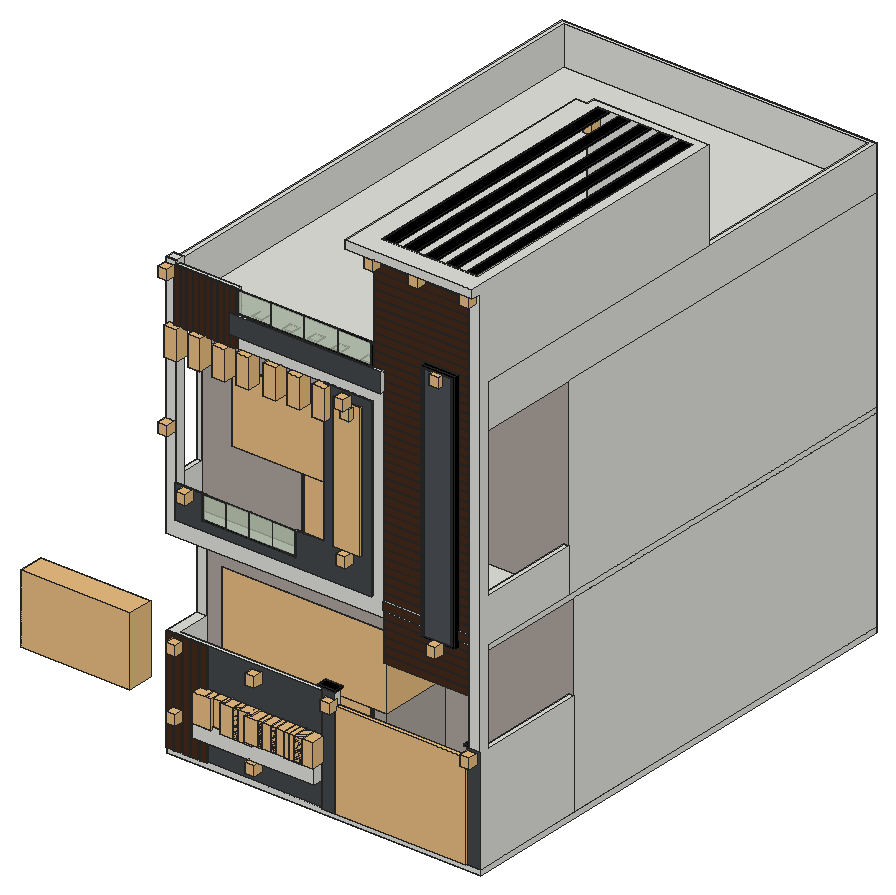
# SketchUp Ruby script. Lengths in inches.
U = 1.inch
M = Sketchup.active_model
def pt(a) = Geom::Point3d.new(a.map { |v| v * U })
def face(e, loops, mat)
  f = e.add_face(loops[0].map { |a| pt(a) })
  loops[1..].each { |l| e.add_face(l.map { |a| pt(a) }).erase! }
  f.material = f.back_material = mat if mat
  f
end
# faces: each face lists its corners as indices into pts; further lists are holes
def faces(e, pts, list, mat = nil) = list.each { |f| face(e, (f[0].is_a?(Array) ? f : [f]).map { |l| l.map { |i| pts[i] } }, mat) }
# xy, xz, yz: faces in a plane at the given z, y or x. An outline is a flat list of corners, or four numbers for a rectangle; further outlines are holes
def ring(l) = l.size == 4 ? [[l[0], l[1]], [l[2], l[1]], [l[2], l[3]], [l[0], l[3]]] : l.each_slice(2).to_a
def flat(e, list, mat, &to3) = list.each { |f| face(e, (f[0].is_a?(Array) ? f : [f]).map { |l| ring(l).map { |u, v| to3.(u, v) } }, mat) }
def xy(e, z, list, mat = nil) = flat(e, list, mat) { |x, y| [x, y, z] }
def xz(e, y, list, mat = nil) = flat(e, list, mat) { |x, z| [x, y, z] }
def yz(e, x, list, mat = nil) = flat(e, list, mat) { |y, z| [x, y, z] }
def lines(e, pts, list) = list.each { |a, b| e.add_line(pt(pts[a]), pt(pts[b])) }
# prism: a flat outline (further loops are holes) pulled along v
def prism(e, loops, v, mat = nil)
  f = face(e, loops, mat); d = Geom::Vector3d.new(v.map { |x| x * U })
  f.pushpull(f.normal.samedirection?(d) ? d.length : -d.length)
end
def box(e, o, s, mat = nil) = prism(e, [[o, [o[0] + s[0], o[1], o[2]], [o[0] + s[0], o[1] + s[1], o[2]], [o[0], o[1] + s[1], o[2]]]], [0, 0, s[2]], mat)
def at(x, y, z, deg = 0) = Geom::Transformation.translation(pt([x, y, z])) * Geom::Transformation.rotation(ORIGIN, Z_AXIS, deg.degrees)
def axes(o, x, y, z) = Geom::Transformation.new([*x, 0, *y, 0, *z, 0, *pt(o).to_a, 1])
def part(name) = M.definitions.add(name)
# library, detail: a bought-in or finely detailed component or shape, given as its bounding box
def library(name, o, s) = part(name).tap { |d| box(d.entities, o, s) }
def detail(e, o, s) = box(e.add_group.entities, o, s)
def put(e, d, t, mat = nil) = e.add_instance(d, t).tap { |i| i.material = mat if mat }
def group(e, t, mat = nil) = e.add_group.tap { |g| g.transformation = t; g.material = mat if mat }.entities
root = M.entities
M.materials.add("Glass Red 001").color = [0, 0, 0]
M.materials["Glass Red 001"].alpha = 0.1
M.materials.add("Glass-Blue manifestation").color = [199, 214, 190]
M.materials["Glass-Blue manifestation"].alpha = 0.52
M.materials.add("Metal - Stainless Steel").color = [215, 211, 217]
M.materials.add("Metal Sandblasted Black 200cm").color = [86, 90, 95]
M.materials.add("Paint - Titanium White").color = [255, 255, 255]
M.materials.add("Tiles Simple H01 100cm").color = [173, 165, 157]
M.materials.add("Wenge Highgloss 300cm").color = [70, 42, 26]
M.materials.add("Wood Black 18-35 80cm").color = [68, 72, 75]
M.materials.add("cnc jali").color = [188, 75, 44]
M.materials.add("glass").color = [255, 255, 255]
M.materials["glass"].alpha = 0.1
M.materials.add("metal").color = [0, 0, 0]
c1 = library("gate 119k",[0,1.18,0],[135.43,4.73,99.21])
c2 = library("Door 01",[-21.26,-2.6,0],[42.52,9.29,84.25])
c3 = library("Hanging Plant 111-02",[-6.97,-7.06,-31.95],[13.94,14.12,31.95])
c4 = library("Scabiosa atropurpurea 005",[-19.05,-18.08,-0.55],[34.7,36.31,33.14])
c5 = library("Skimmia japonica Rubella 004",[-17.08,-16.64,-0.26],[33.2,34.59,28.81])
c6 = library("Spot Light",[-5.1,-5.1,-11.05],[10.2,10.2,11.05])
c7 = library("Spot Light\#1",[-5.1,-5.1,-11.05],[10.2,10.2,11.05])
c8 = library("Spot Light\#2",[-5.1,-5.1,-11.05],[10.2,10.2,11.05])
c9 = library("Spot Light\#3",[-5.1,-5.1,-11.05],[10.2,10.2,11.05])
c10 = library("Spot Light\#4",[-5.1,-5.1,-11.05],[10.2,10.2,11.05])
c11 = library("Spot Light\#5",[-5.1,-5.1,-11.05],[10.2,10.2,11.05])
c12 = library("Spot Light\#6",[-5.1,-5.1,-11.05],[10.2,10.2,11.05])
c13 = library("Spot Light\#7",[-5.1,-5.1,-11.05],[10.2,10.2,11.05])
c14 = library("Spot Light\#8",[-5.1,-5.1,-11.05],[10.2,10.2,11.05])
c15 = library("Spot Light\#9",[-5.1,-5.1,-11.05],[10.2,10.2,11.05])
c16 = library("Spot Light\#10",[-5.1,-5.1,-11.05],[10.2,10.2,11.05])
c17 = library("Spot Light\#11",[-5.1,-5.1,-11.05],[10.2,10.2,11.05])
c18 = library("Spot Light\#13",[-5.1,-5.1,-11.05],[10.2,10.2,11.05])
c19 = library("Spot Light\#15",[-5.1,-5.1,-11.05],[10.2,10.2,11.05])
c20 = library("Spot Light\#16",[-5.1,-5.1,-11.05],[10.2,10.2,11.05])
c21 = library("Spot Light\#17",[-5.1,-5.1,-11.05],[10.2,10.2,11.05])
c22 = library("Spot Light\#18",[-5.1,-5.1,-11.05],[10.2,10.2,11.05])
c23 = library("Spot Light\#19",[-5.1,-5.1,-11.05],[10.2,10.2,11.05])
c24 = library("Spot Light\#20",[-5.1,-5.1,-11.05],[10.2,10.2,11.05])
c25 = library("Spot Light\#21",[-5.1,-5.1,-11.05],[10.2,10.2,11.05])
c26 = library("Spot Light\#22",[-5.1,-5.1,-11.05],[10.2,10.2,11.05])
c27 = library("Spot Light\#23",[-5.1,-5.1,-11.05],[10.2,10.2,11.05])
c28 = library("Spot Light\#24",[-5.1,-5.1,-11.05],[10.2,10.2,11.05])
c29 = library("Spot Light\#25",[-5.1,-5.1,-11.05],[10.2,10.2,11.05])
c30 = library("Spot Light\#26",[-5.1,-5.1,-11.05],[10.2,10.2,11.05])
c31 = library("Spot Light\#27",[-5.1,-5.1,-11.05],[10.2,10.2,11.05])
c32 = library("Spot Light\#28",[-5.1,-5.1,-11.05],[10.2,10.2,11.05])
c33 = library("Spot Light\#31",[-5.1,-5.1,-11.05],[10.2,10.2,11.05])
c34 = library("Spot Light\#34",[-5.1,-5.1,-11.05],[10.2,10.2,11.05])
c35 = library("Spot Light\#37",[-5.1,-5.1,-11.05],[10.2,10.2,11.05])
c36 = library("Spot Light\#38",[-5.1,-5.1,-11.05],[10.2,10.2,11.05])
c37 = library("Spot Light\#41",[-5.1,-5.1,-11.05],[10.2,10.2,11.05])
c38 = library("Spot Light\#42",[-5.1,-5.1,-11.05],[10.2,10.2,11.05])
c39 = library("Spot Light\#43",[-5.1,-5.1,-11.05],[10.2,10.2,11.05])
c40 = library("Spot Light\#44",[-5.1,-5.1,-11.05],[10.2,10.2,11.05])
c41 = library("Spot Light\#45",[-5.1,-5.1,-11.05],[10.2,10.2,11.05])
c42 = library("Dome Light",[-12,-12,0],[24,24,12])
c43 = library("Group\#12",[-13.12,-1.5,-18.99],[144.1,102,79.93])
c44 = library("Group\#14",[0,-3,0],[100.03,34.78,78.78])
c45 = part("Group\#41")
box(c45.entities,[0,0,-2],[9.86,293.9375,2])
c46 = library("Group\#43",[0,0,0],[48,96,0.5])
c47 = part("Group758")
box(c47.entities,[275.39,542.01,104.72],[1.97,4.92,1.97],"Metal - Stainless Steel")
c48 = part("Group760")
box(c48.entities,[173.03,542.01,146.0625],[1.97,4.92,1.97],"Metal - Stainless Steel")
c49 = part("Group761")
box(c49.entities,[275.39,542.01,146.0625],[1.97,4.92,1.97],"Metal - Stainless Steel")
c50 = part("Group755")
box(c50.entities,[199.8,545.35,104.72],[25,1.19,43.31],"Glass-Blue manifestation")
c51 = part("Group753")
xy(c51.entities,106.69,[[174.61,545.35,199.02,546.54]],"Paint - Titanium White")
xy(c51.entities,146.0625,[[174.61,545.35,199.02,546.54]],"Paint - Titanium White")
xz(c51.entities,545.35,[[174.61,106.69,199.02,146.0625]],"Glass-Blue manifestation")
xz(c51.entities,546.54,[[174.61,106.69,199.02,146.0625]],"Glass-Blue manifestation")
yz(c51.entities,174.61,[[545.35,106.69,546.54,146.0625]],"Paint - Titanium White")
yz(c51.entities,199.02,[[545.35,106.69,546.54,146.0625]],"Glass-Blue manifestation")
c52 = part("Group756")
xy(c52.entities,106.69,[[251.38,545.35,275.79,546.54]],"Paint - Titanium White")
xy(c52.entities,146.0625,[[251.38,545.35,275.79,546.54]],"Paint - Titanium White")
xz(c52.entities,545.35,[[251.38,106.69,275.79,146.0625]],"Glass-Blue manifestation")
xz(c52.entities,546.54,[[251.38,106.69,275.79,146.0625]],"Glass-Blue manifestation")
yz(c52.entities,251.38,[[545.35,106.69,546.54,146.0625]],"Glass-Blue manifestation")
yz(c52.entities,275.79,[[545.35,106.69,546.54,146.0625]],"Paint - Titanium White")
c53 = part("Group754")
box(c53.entities,[225.59,545.35,104.72],[25,1.19,43.31],"Glass-Blue manifestation")
c54 = part("Group757")
box(c54.entities,[173.03,542.01,104.72],[1.97,4.92,1.97],"Metal - Stainless Steel")
c55 = part("Group751\#1")
box(c55.entities,[173.43,542.01,106.69],[1.18,4.53,39.37],"metal")
c56 = part("Group762\#1")
box(c56.entities,[175,544.96,146.0625],[100.39,1.97,1.97],"metal")
c57 = part("Group752\#1")
box(c57.entities,[275.79,542.01,106.69],[1.18,4.53,39.37],"metal")
c58 = part("Group759\#1")
box(c58.entities,[175,544.96,104.72],[100.39,1.97,1.97],"metal")
xy(root,0,[[170.625,10,170.625,12,0,12,0,61.5,196.875,61.5,196.875,141,241.875,141,241.875,132,208.125,132,208.125,52.5,11.25,52.5,11.25,16.5,185.625,16.5,185.625,10],[328.2,12,328.2,21,337.58,21,337.58,139.5,343.125,139.5,343.125,12]])
xy(root,9.99,[[114.7,52.5,193.21,61.5]])
xy(root,107.29,[[45.15,52.5,99.05,61.5]])
xy(root,114,[[0,12,170.625,12,170.625,16.5,11.25,16.5,11.25,52.375,0,52.375],[337.58,21,343.125,139.5]])
xy(root,115.74,[[331.95,10,343.125,12],[328.2,12,331.95,21]])
xy(root,120,[[170.625,10,185.625,16.5]])
xy(root,167.55,[[114.7,52.5,193.21,61.5]])
xy(root,168.22,[[45.15,52.5,99.05,61.5]])
xy(root,209.75,[[0,52.375,11.25,52.375,11.25,52.5,208.125,52.5,208.125,132,241.875,132,241.875,141,196.875,141,196.875,61.5,0,61.5]])
xy(root,215.75,[[238.2,10,238.2,12,0,12,0,61.5,196.875,61.5,196.875,141,241.875,141,241.875,132,208.125,132,208.125,52.5,5.625,52.5,5.625,21,11.25,21,11.25,16.5,331.95,16.5,331.95,10],[337.58,21,343.125,132]])
xy(root,225.12,[[114.7,52.5,193.21,61.5]])
xy(root,227.5625,[[238.2,10,331.95,10,331.95,16.5,11.25,16.5,11.25,12,238.2,12]])
xy(root,263.5625,[[0,21,5.625,52.375]])
xy(root,263.73,[[337.58,21,343.125,132]])
xy(root,292.18,[[41.11,52.5,101.97,61.5]])
xy(root,370.96,[[41.11,52.5,101.97,61.5]])
xy(root,377.18,[[114.7,52.5,193.21,61.5]])
xy(root,425.5,[[0,52.375,5.625,52.375,5.625,52.5,208.125,52.5,208.125,132,241.875,132,241.875,141,196.875,141,196.875,61.5,0,61.5]])
xy(root,431.5,[[216.95,314.9375,228.2,323.9375]])
xy(root,473.5,[[331.875,21,331.875,314.9375,228.2,314.9375,228.2,323.9375,343.125,323.9375,343.125,21]])
xy(root,479.5,[[0,12,11.25,21]])
xy(root,563.5,[[204.45,0,204.45,314.9375,228.2,314.9375,228.2,21,331.95,21,331.95,10,343.125,10,343.125,0]])
xy(root,572.5,[[[204.45,0,343.125,0,343.125,323.9375,216.95,323.9375,216.95,314.9375,204.45,314.9375],[228.2,21,331.875,314.9375]]])
xz(root,0,[[204.45,563.5,343.125,572.5]])
xz(root,10,[[331.95,115.74,343.125,115.74,343.125,563.5,331.95,563.5,331.95,227.5625,238.2,227.5625,238.2,215.75,331.95,215.75]])
xz(root,10,[[170.625,0,185.625,120]],"Wood Black 18-35 80cm")
xz(root,12,[[0,0,45,0,45,27,170.625,27,170.625,45,45,45,45,114,0,114],[0,209.75,238.2,215.75],[0,215.75,238.2,215.75,238.2,227.5625,11.25,227.5625,11.25,479.5,0,479.5]])
xz(root,12,[[45,0,170.625,27],[328.2,0,343.125,115.74],[45,45,170.625,114]],"Wood Black 18-35 80cm")
xz(root,16.5,[[11.25,0,11.25,114,170.625,114,170.625,120,185.625,120,185.625,0],[11.25,215.75,331.95,227.5625]])
xz(root,21,[[328.2,0,328.2,115.74,331.95,115.74,331.95,227.5625,337.58,227.5625,337.58,215.75,343.125,215.75,343.125,114,337.58,114,337.58,0],[5.625,215.75,11.25,227.5625],[5.625,227.5625,5.625,263.5625,0,263.5625,0,479.5,11.25,479.5,11.25,227.5625],[331.95,227.5625,331.95,473.5,343.125,473.5,343.125,263.73,337.58,263.73,337.58,227.5625],[331.875,473.5,331.95,563.5],
  [228.2,563.5,331.875,572.5]])
xz(root,52.375,[[0,114,11.25,209.75],[0,263.5625,5.625,425.5]])
xz(root,52.5,[[[11.25,0,208.125,209.75],[114.7,9.99,193.21,167.55],[45.15,107.29,99.05,168.22]],[[5.625,215.75,208.125,425.5],[114.7,225.12,193.21,377.18],[41.11,292.18,101.97,370.96]]],"Tiles Simple H01 100cm")
xz(root,61.5,[[[0,0,196.875,209.75],[114.7,9.99,193.21,167.55],[45.15,107.29,99.05,168.22]],[[0,215.75,196.875,425.5],[114.7,225.12,193.21,377.18],[41.11,292.18,101.97,370.96]]])
xz(root,132,[[337.58,215.75,343.125,263.73]])
xz(root,132,[[208.125,0,241.875,209.75],[208.125,215.75,241.875,425.5]],"Tiles Simple H01 100cm")
xz(root,139.5,[[337.58,0,343.125,114]])
xz(root,141,[[196.875,0,241.875,209.75],[196.875,215.75,241.875,425.5]])
xz(root,314.9375,[[216.95,431.5,228.2,431.5,228.2,473.5,331.875,473.5,331.875,572.5,228.2,572.5,228.2,563.5,216.95,563.5],[204.45,563.5,216.95,572.5]])
xz(root,323.9375,[[216.95,431.5,216.95,572.5,343.125,572.5,343.125,473.5,228.2,473.5,228.2,431.5]])
yz(root,0,[[12,0,12,114,52.375,114,52.375,209.75,61.5,209.75,61.5,0],[12,215.75,12,479.5,21,479.5,21,263.5625,52.375,263.5625,52.375,425.5,61.5,425.5,61.5,215.75]])
yz(root,5.625,[[21,215.75,52.5,215.75,52.5,425.5,52.375,425.5,52.375,263.5625,21,263.5625]])
yz(root,11.25,[[16.5,0,52.5,0,52.5,209.75,52.375,209.75,52.375,114,16.5,114],[16.5,215.75,21,215.75,21,479.5,12,479.5,12,227.5625,16.5,227.5625]])
yz(root,41.11,[[52.5,292.18,61.5,370.96]])
yz(root,45.15,[[52.5,107.29,61.5,168.22]])
yz(root,99.05,[[52.5,107.29,61.5,168.22]])
yz(root,101.97,[[52.5,292.18,61.5,370.96]])
yz(root,114.7,[[52.5,9.99,61.5,167.55],[52.5,225.12,61.5,377.18]])
yz(root,170.625,[[10,114,16.5,120]])
yz(root,170.625,[[10,0,12,114]],"Wood Black 18-35 80cm")
yz(root,185.625,[[10,0,16.5,120]])
yz(root,193.21,[[52.5,9.99,61.5,167.55],[52.5,225.12,61.5,377.18]])
yz(root,196.875,[[61.5,0,141,209.75],[61.5,215.75,141,425.5]])
yz(root,204.45,[[0,563.5,314.9375,572.5]])
yz(root,208.125,[[52.5,0,132,209.75],[52.5,215.75,132,425.5]],"Tiles Simple H01 100cm")
yz(root,216.95,[[314.9375,431.5,323.9375,572.5]])
yz(root,228.2,[[314.9375,431.5,323.9375,473.5],[21,563.5,314.9375,572.5]])
yz(root,238.2,[[10,215.75,12,227.5625]])
yz(root,241.875,[[132,215.75,141,425.5]])
yz(root,241.875,[[132,0,141,209.75]],"Tiles Simple H01 100cm")
yz(root,328.2,[[12,0,21,115.74]])
yz(root,331.875,[[21,473.5,314.9375,572.5]])
yz(root,331.95,[[10,115.74,10,215.75,16.5,215.75,16.5,227.5625,10,227.5625,10,563.5,21,563.5,21,115.74]])
yz(root,337.58,[[21,0,139.5,114],[21,215.75,132,263.73]])
yz(root,343.125,[[12,0,139.5,0,139.5,114,21,114,21,215.75,132,215.75,132,263.73,21,263.73,21,473.5,323.9375,473.5,323.9375,572.5,0,572.5,0,563.5,10,563.5,10,115.74,12,115.74]])
put(root,c1,axes([185.625,8.82,0],[1.05276,0,0],[0,1,0],[0,0,1.06]))
put(root,c2,axes([154.15,53.7,12.91],[1.72,0,0],[0,-0.18,0],[0,0,1.81178]))
put(root,c2,axes([154.15,54.58,229.59],[1.72,0,0],[0,-0.3102,0],[0,0,1.728]))
put(root,c3,at(174.45,8.27,418.3125))
put(root,c3,at(145.06,10,418.3125))
put(root,c3,at(119.1,10,418.3125))
put(root,c3,at(89.6875,10,418.3125))
put(root,c3,at(65.17,8,418.3125))
put(root,c3,at(38.41,8,419.53))
put(root,c3,at(11.25,10,418.3125))
put(root,c4,axes([49.14,6.58,42.07],[0.59323,0,0],[0,0.39156,0],[0,0,0.92207]))
put(root,c4,axes([62.56,8.58,42.07],[0.59323,0,0],[0,0.39156,0],[0,0,0.92207]))
put(root,c4,axes([79,6.31,41.92],[0.59323,0,0],[0,0.39156,0],[0,0,0.92207]))
put(root,c4,axes([93.5,6.31,41.92],[0.59323,0,0],[0,0.39156,0],[0,0,0.92207]))
put(root,c5,axes([107.87,10.93,46.18],[0.5984,0,0],[0,0.93086,0],[0,0,0.88]))
put(root,c5,axes([122.37,10.93,46.18],[0.5984,0,0],[0,0.93086,0],[0,0,0.88]))
put(root,c5,axes([136.93,10.93,46.18],[0.5984,0,0],[0,0.93086,0],[0,0,0.88]))
put(root,c5,axes([151.56,10.93,46.18],[0.5984,0,0],[0,0.93086,0],[0,0,0.88]))
put(root,c5,axes([162.77,10.93,46.18],[0.5984,0,0],[0,0.93086,0],[0,0,0.88]))
put(root,c6,at(16.93,46.3,431.49))
put(root,c7,at(45.4,46.5625,431.49))
put(root,c8,at(73.89,47.78,431.49))
put(root,c9,at(107.61,47.14,431.49))
put(root,c10,at(134.68,47.75,431.49))
put(root,c11,at(161.69,47.04,431.49))
put(root,c12,at(193.04,46.72,431.49))
put(root,c13,at(212.2,123.22,431.49))
put(root,c14,at(327.08,116.81,431.49))
put(root,c15,at(324.72,36.13,431.49))
put(root,c16,at(202.63,19.16,431.49))
put(root,c17,at(7.22,34.64,209.74))
put(root,c18,at(104.86,40.03,209.74))
put(root,c19,at(198.76,38.24,209.74))
put(root,c20,at(215.8,113.33,209.74))
put(root,c21,at(310.91,116.95,209.74))
put(root,c22,at(315.02,24.69,209.74))
put(root,c23,at(253.14,28.97,209.74))
put(root,c24,at(230.18,4.22,563.49))
put(root,c25,at(278.23,5.24,563.49))
put(root,c26,at(334,5.05,563.49))
put(root,c27,at(217.54,32.32,563.49))
put(root,c28,at(211.89,112.68,563.49))
put(root,c29,at(213.52,210.58,563.49))
put(root,c30,at(228.2,306.28,563.49))
put(root,c31,at(103.98,0,27))
put(root,c32,at(103.98,0,113.79))
put(root,c33,at(301.88,-0.2,211.79))
put(root,c34,at(13.5625,4.9,110.46))
put(root,c35,at(333.31,6.9,111.7))
put(root,c36,at(301.88,4.19,474.41))
put(root,c37,at(5.1,4.9,322.9375))
put(root,c38,at(202.37,6.55,406.27))
put(root,c39,at(200.15,1.45,417.5))
put(root,c40,at(200.7,3.16,263.49))
put(root,c41,at(26.25,3.16,263.55))
put(root,c35,at(180.7,6.9,111.7))
put(root,c34,at(13.5625,4.9,42.71))
put(root,c37,at(6.15,2.9,476.55))
put(root,c42,axes([-109.63,38.04,32.55],[5,0,0],[0,-1.17,0],[0,0,6.24]))
g1 = group(root,at(0,132,0))
box(g1,[95.625,214.5,0],[5.625,12,209.75])
prism(g1,[[[166.875,358.5,0],[166.875,363,0],[266.25,363,0],[266.25,375,0],[271.875,375,0],[271.875,358.5,0]]],[0,0,209.75])
xy(g1,0,[[11.25,174,101.25,178.5]])
xy(g1,209.75,[[0,-70.5,11.25,-70.5,11.25,411,331.86,410.99,331.86,8.99,316.71,8.99,316.71,-0.01,343.11,-0.01,343.11,410.99,343.125,420,0,420],[11.25,174,101.25,178.5]])
xz(g1,174,[[11.25,0,101.25,209.75]])
xz(g1,178.5,[[11.25,0,101.25,209.75]])
yz(g1,11.25,[[174,0,178.5,209.75]])
yz(g1,101.25,[[174,0,178.5,209.75]])
g2 = group(g1,at(0,0,0))
xy(g2,0,[[11.25,226.5,116.25,231],[161.25,226.5,286.875,226.5,286.875,231,166.875,231,166.875,411,161.25,411]])
xy(g2,209.75,[[11.25,226.5,116.25,231],[161.25,226.5,286.875,226.5,286.875,231,166.875,231,166.875,411,161.25,411]])
xz(g2,-70.5,[[5.625,0,11.25,209.75]])
xz(g2,7.5,[[242.03,-0.04,332.03,0,343.125,0,343.125,209.75,316.72,209.74,241.87,209.71]],"Tiles Simple H01 100cm")
xz(g2,9,[[242.03,-0.04,241.87,209.71,316.72,209.74,331.875,209.75,331.875,0],[331.875,0,331.875,209.75,332.03,0]])
xz(g2,226.5,[[11.25,0,116.25,209.75],[161.25,0,286.875,209.75]])
xz(g2,231,[[11.25,0,116.25,209.75],[166.875,0,286.875,209.75]])
xz(g2,411,[[11.25,0,161.25,209.75],[161.25,0,166.875,209.75],[166.875,0,331.875,209.75]])
xz(g2,420,[[0,0,343.125,209.75]])
yz(g2,0,[[-70.5,0,420,209.75]])
yz(g2,11.25,[[-70.5,0,226.5,209.75],[226.5,0,231,209.75],[231,0,411,209.75]])
yz(g2,116.25,[[226.5,0,231,209.75]])
yz(g2,161.25,[[226.5,0,411,209.75]])
yz(g2,166.875,[[231,0,411,209.75]])
yz(g2,286.875,[[226.5,0,231,209.75]])
yz(g2,331.875,[[9,0,411,209.75]])
yz(g2,343.125,[[7.5,0,420,209.75]])
p = [[242.03,7.5,-0.04],[241.87,7.5,209.71],[241.87,9,209.71],[242.03,9,-0.04],[332.03,9,0],[332.03,7.5,0],
  [331.875,9,0],[316.72,7.5,209.74],[316.72,9,209.74]]
faces(g2,p,[[0,1,2,3],[4,5,0,3,6],[7,8,2,1]])
g3 = group(g2,at(5.625,-115.5,0))
xy(g3,-6,[[-5.625,-4.5,-5.625,342,110.625,342,110.625,346.5,-5.625,346.5,-5.625,535.5,155.625,535.5,155.625,342,281.25,342,281.25,346.5,161.25,346.5,161.25,535.5,337.5,535.5,337.5,-4.5],[-5.625,342,110.625,346.5],[155.625,342,155.625,535.5,161.25,535.5,161.25,346.5,281.25,346.5,281.25,342]])
xy(g3,0,[[-5.625,-4.5,337.5,-4.5,337.5,535.5,161.25,535.5,161.25,346.5,281.25,346.5,281.25,342,155.625,342,155.625,535.5,-5.625,535.5,-5.625,346.5,110.625,346.5,110.625,342,-5.625,342],[-5.625,342,110.625,346.5],[155.625,342,281.25,342,281.25,346.5,161.25,346.5,161.25,535.5,155.625,535.5]])
xz(g3,-4.5,[[-5.625,-6,337.5,0]])
xz(g3,342,[[-5.625,-6,110.625,0],[155.625,-6,281.25,0]])
xz(g3,346.5,[[-5.625,-6,110.625,0],[161.25,-6,281.25,0]])
xz(g3,535.5,[[-5.625,-6,155.625,0],[155.625,-6,161.25,0],[161.25,-6,337.5,0]])
yz(g3,-5.625,[[-4.5,-6,342,0],[342,-6,346.5,0],[346.5,-6,535.5,0]])
yz(g3,110.625,[[342,-6,346.5,0]])
yz(g3,155.625,[[342,-6,535.5,0]])
yz(g3,161.25,[[346.5,-6,535.5,0]])
yz(g3,281.25,[[342,-6,346.5,0]])
yz(g3,337.5,[[-4.5,-6,535.5,0]])
g4 = group(root,at(0,12,0))
xz(g4,0,[[0,0,45,114]])
g5 = group(root,at(0,12,0),"Wenge Highgloss 300cm")
xy(g5,0,[[0,-2,7.67,0]])
xy(g5,114,[[0,-2,7.67,0]])
xz(g5,-2,[[0,0,7.67,114]],"Wenge Highgloss 300cm")
xz(g5,0,[[0,0,7.67,114]],"Wenge Highgloss 300cm")
yz(g5,0,[[-2,0,0,114]],"Wenge Highgloss 300cm")
yz(g5,7.67,[[-2,0,0,114]],"Wenge Highgloss 300cm")
g6 = group(root,at(9.33,12,0),"Wenge Highgloss 300cm")
xy(g6,0,[[0,-2,7.67,0]])
xy(g6,114,[[0,-2,7.67,0]])
xz(g6,-2,[[0,0,7.67,114]],"Wenge Highgloss 300cm")
xz(g6,0,[[0,0,7.67,114]],"Wenge Highgloss 300cm")
yz(g6,0,[[-2,0,0,114]],"Wenge Highgloss 300cm")
yz(g6,7.67,[[-2,0,0,114]],"Wenge Highgloss 300cm")
g7 = group(root,at(18.67,12,0),"Wenge Highgloss 300cm")
xy(g7,0,[[0,-2,7.67,0]])
xy(g7,114,[[0,-2,7.67,0]])
xz(g7,-2,[[0,0,7.67,114]],"Wenge Highgloss 300cm")
xz(g7,0,[[0,0,7.67,114]],"Wenge Highgloss 300cm")
yz(g7,0,[[-2,0,0,114]],"Wenge Highgloss 300cm")
yz(g7,7.67,[[-2,0,0,114]],"Wenge Highgloss 300cm")
g8 = group(root,at(28,12,0),"Wenge Highgloss 300cm")
xy(g8,0,[[0,-2,7.67,0]])
xy(g8,114,[[0,-2,7.67,0]])
xz(g8,-2,[[0,0,7.67,114]],"Wenge Highgloss 300cm")
xz(g8,0,[[0,0,7.67,114]],"Wenge Highgloss 300cm")
yz(g8,0,[[-2,0,0,114]],"Wenge Highgloss 300cm")
yz(g8,7.67,[[-2,0,0,114]],"Wenge Highgloss 300cm")
g9 = group(root,at(37.33,12,0),"Wenge Highgloss 300cm")
xy(g9,0,[[0,-2,7.67,0]])
xy(g9,114,[[0,-2,7.67,0]])
xz(g9,-2,[[0,0,7.67,114]],"Wenge Highgloss 300cm")
xz(g9,0,[[0,0,7.67,114]],"Wenge Highgloss 300cm")
yz(g9,0,[[-2,0,0,114]],"Wenge Highgloss 300cm")
yz(g9,7.67,[[-2,0,0,114]],"Wenge Highgloss 300cm")
g10 = group(root,at(45,12,27))
xy(g10,0,[[-7.67,-12,125.625,0]])
xy(g10,1,[[-5.17,-10,123.125,-2.3125]])
xy(g10,18,[[[-7.67,-12,125.625,0],[-5.17,-10,123.125,-2.3125]]])
xz(g10,-12,[[-7.67,0,125.625,18]])
xz(g10,-10,[[-5.17,1,123.125,18]])
xz(g10,-2.3125,[[-5.17,1,123.125,18]])
xz(g10,0,[[-7.67,0,125.625,18]])
yz(g10,-7.67,[[-12,0,0,18]])
yz(g10,-5.17,[[-10,1,-2.3125,18]])
yz(g10,123.125,[[-10,1,-2.3125,18]])
yz(g10,125.625,[[-12,0,0,18]])
put(root,c43,axes([45.15,52.5,107.29],[1.25,0,0],[0,1,0],[0,0,1]))
put(root,c44,axes([41.11,52.5,292.18],[1.25,0,0],[0,1,0],[0,0,1]))
g11 = group(root,at(114.7,52.5,225.12))
prism(g11,[[[78.52,0,0],[78.52,0,152.0625],[0,0,152.0625],[0,0,0]],[[2.5,0,150.0625],[76.02,0,150.0625],[76.02,0,2],[2.5,0,2]]],[0,2.5,0],"metal")
g12 = group(root,at(114.7,52.5,9.99),"metal")
prism(g12,[[[78.52,0,0],[78.52,0,157.5625],[0,0,157.5625],[0,0,0]],[[76.02,0,155.5625],[76.02,0,2],[2.5,0,2],[2.5,0,155.5625]]],[0,2.5,0])
g13 = group(root,at(11.25,12,227.5625))
prism(g13,[[[0,0,251.9375],[0,0,203.9375],[226.95,0,203.9375],[226.95,0,-17.8125],[-11.25,0,-17.8125],[-11.25,0,251.9375]],[[215.7,0,190.75],[0,0,190.75],[0,0,0],[215.7,0,0]]],[0,-2,0])
g14 = group(g13,at(0,-3.73,0))
prism(g14,[[[215.7,1.73,0],[0,1.73,0],[0,1.73,36],[30,1.73,36],[30,1.73,9],[133.2,1.73,9],[133.2,1.73,36],[163.2,1.73,36],[163.2,1.73,190.75],[215.7,1.73,190.75]],[[174.45,1.73,35.9375],[204.45,1.73,35.9375],[204.45,1.73,181.75],[174.45,1.73,181.75]]],[0,-1.73,0],"Wood Black 18-35 80cm")
g15 = group(root,at(238.2,12,434.38))
box(g15,[0,0.75,-268.0625],[93.75,1.25,397.04])
g16 = group(root,at(238.2,12,555.58),"Wenge Highgloss 300cm")
box(g16,[-10,-2,0],[103.75,2,7.78],"Wenge Highgloss 300cm")
g17 = group(root,at(238.2,12,546.93),"Wenge Highgloss 300cm")
box(g17,[-10,-2,0],[103.75,2,7.78],"Wenge Highgloss 300cm")
g18 = group(root,at(238.2,12,538.28),"Wenge Highgloss 300cm")
box(g18,[-10,-2,0],[103.75,2,7.78],"Wenge Highgloss 300cm")
g19 = group(root,at(238.2,12,529.625),"Wenge Highgloss 300cm")
box(g19,[-10,-2,0],[103.75,2,7.78],"Wenge Highgloss 300cm")
g20 = group(root,at(238.2,12,520.98),"Wenge Highgloss 300cm")
box(g20,[-10,-2,0],[103.75,2,7.78],"Wenge Highgloss 300cm")
g21 = group(root,at(238.2,12,512.33),"Wenge Highgloss 300cm")
box(g21,[-10,-2,0],[103.75,2,7.78],"Wenge Highgloss 300cm")
g22 = group(root,at(238.2,12,503.68),"Wenge Highgloss 300cm")
box(g22,[-10,-2,0],[103.75,2,7.78],"Wenge Highgloss 300cm")
g23 = group(root,at(238.2,12,495.03),"Wenge Highgloss 300cm")
box(g23,[-10,-2,0],[103.75,2,7.78],"Wenge Highgloss 300cm")
g24 = group(root,at(238.2,12,486.375),"Wenge Highgloss 300cm")
box(g24,[-10,-2,0],[103.75,2,7.78],"Wenge Highgloss 300cm")
g25 = group(root,at(238.2,12,477.73),"Wenge Highgloss 300cm")
box(g25,[-10,-2,0],[103.75,2,7.78],"Wenge Highgloss 300cm")
g26 = group(root,at(238.2,12,469.08),"Wenge Highgloss 300cm")
box(g26,[-10,-2,0],[103.75,2,7.78],"Wenge Highgloss 300cm")
g27 = group(root,at(238.2,12,460.42),"Wenge Highgloss 300cm")
box(g27,[-10,-2,0],[103.75,2,7.78],"Wenge Highgloss 300cm")
g28 = group(root,at(238.2,12,451.77),"Wenge Highgloss 300cm")
box(g28,[-10,-2,0],[103.75,2,7.78],"Wenge Highgloss 300cm")
g29 = group(root,at(238.2,12,443.125),"Wenge Highgloss 300cm")
box(g29,[-10,-2,0],[103.75,2,7.78],"Wenge Highgloss 300cm")
g30 = group(root,at(238.2,12,434.47),"Wenge Highgloss 300cm")
box(g30,[-10,-2,0],[103.75,2,7.78],"Wenge Highgloss 300cm")
g31 = group(root,at(238.2,12,425.82),"Wenge Highgloss 300cm")
box(g31,[0,-2,0],[93.75,2,7.78],"Wenge Highgloss 300cm")
g32 = group(root,at(238.2,12,417.17),"Wenge Highgloss 300cm")
box(g32,[0,-2,0],[93.75,2,7.78],"Wenge Highgloss 300cm")
g33 = group(root,at(238.2,12,408.52),"Wenge Highgloss 300cm")
box(g33,[0,-2,0],[93.75,2,7.78],"Wenge Highgloss 300cm")
g34 = group(root,at(238.2,12,399.875),"Wenge Highgloss 300cm")
box(g34,[0,-2,0],[93.75,2,7.78],"Wenge Highgloss 300cm")
g35 = group(root,at(238.2,12,391.22),"Wenge Highgloss 300cm")
box(g35,[0,-2,0],[93.75,2,7.78],"Wenge Highgloss 300cm")
g36 = group(root,at(238.2,12,382.57),"Wenge Highgloss 300cm")
box(g36,[0,-2,0],[93.75,2,7.78],"Wenge Highgloss 300cm")
g37 = group(root,at(238.2,12,373.92),"Wenge Highgloss 300cm")
box(g37,[0,-2,0],[93.75,2,7.78],"Wenge Highgloss 300cm")
g38 = group(root,at(238.2,12,365.27),"Wenge Highgloss 300cm")
box(g38,[0,-2,0],[93.75,2,7.78],"Wenge Highgloss 300cm")
g39 = group(root,at(238.2,12,356.62),"Wenge Highgloss 300cm")
box(g39,[0,-2,0],[93.75,2,7.78],"Wenge Highgloss 300cm")
g40 = group(root,at(238.2,12,347.97),"Wenge Highgloss 300cm")
box(g40,[0,-2,0],[93.75,2,7.78],"Wenge Highgloss 300cm")
g41 = group(root,at(238.2,12,339.32),"Wenge Highgloss 300cm")
box(g41,[0,-2,0],[93.75,2,7.78],"Wenge Highgloss 300cm")
g42 = group(root,at(238.2,12,330.67),"Wenge Highgloss 300cm")
box(g42,[0,-2,0],[93.75,2,7.78],"Wenge Highgloss 300cm")
g43 = group(root,at(238.2,12,322.02),"Wenge Highgloss 300cm")
box(g43,[0,-2,0],[93.75,2,7.78],"Wenge Highgloss 300cm")
g44 = group(root,at(238.2,12,313.37),"Wenge Highgloss 300cm")
box(g44,[0,-2,0],[93.75,2,7.78],"Wenge Highgloss 300cm")
g45 = group(root,at(238.2,12,304.72),"Wenge Highgloss 300cm")
box(g45,[0,-2,0],[93.75,2,7.78],"Wenge Highgloss 300cm")
g46 = group(root,at(238.2,12,296.07),"Wenge Highgloss 300cm")
box(g46,[0,-2,0],[93.75,2,7.78],"Wenge Highgloss 300cm")
g47 = group(root,at(238.2,12,287.42),"Wenge Highgloss 300cm")
box(g47,[0,-2,0],[93.75,2,7.78],"Wenge Highgloss 300cm")
g48 = group(root,at(238.2,12,278.77),"Wenge Highgloss 300cm")
box(g48,[0,-2,0],[93.75,2,7.78],"Wenge Highgloss 300cm")
g49 = group(root,at(238.2,12,270.12),"Wenge Highgloss 300cm")
box(g49,[0,-2,0],[93.75,2,7.78],"Wenge Highgloss 300cm")
g50 = group(root,at(238.2,12,261.47),"Wenge Highgloss 300cm")
box(g50,[0,-2,0],[93.75,2,7.78],"Wenge Highgloss 300cm")
g51 = group(root,at(238.2,12,252.82),"Wenge Highgloss 300cm")
box(g51,[0,-2,0],[93.75,2,7.78],"Wenge Highgloss 300cm")
g52 = group(root,at(238.2,12,244.17),"Wenge Highgloss 300cm")
box(g52,[0,-2,0],[93.75,2,7.78],"Wenge Highgloss 300cm")
g53 = group(root,at(238.2,12,235.52),"Wenge Highgloss 300cm")
box(g53,[0,-2,0],[93.75,2,7.78],"Wenge Highgloss 300cm")
g54 = group(root,at(238.2,12,226.87),"Wenge Highgloss 300cm")
box(g54,[0,-2,0],[93.75,2,7.78],"Wenge Highgloss 300cm")
g55 = group(root,at(238.2,12,218.22),"Wenge Highgloss 300cm")
box(g55,[0,-3.1875,0],[93.75,3.1875,7.78],"Wenge Highgloss 300cm")
g56 = group(root,at(238.2,12,209.57),"Wenge Highgloss 300cm")
box(g56,[0,-2,0],[93.75,2,7.78],"Wenge Highgloss 300cm")
g57 = group(root,at(238.2,12,200.92),"Wenge Highgloss 300cm")
box(g57,[0,-2,0],[93.75,2,7.78],"Wenge Highgloss 300cm")
g58 = group(root,at(238.2,12,192.27),"Wenge Highgloss 300cm")
box(g58,[0,-2,0],[93.75,2,7.78],"Wenge Highgloss 300cm")
g59 = group(root,at(238.2,12,183.62),"Wenge Highgloss 300cm")
box(g59,[0,-2,0],[93.75,2,7.78],"Wenge Highgloss 300cm")
g60 = group(root,at(238.2,12,174.97),"Wenge Highgloss 300cm")
box(g60,[0,-2,0],[93.75,2,7.78],"Wenge Highgloss 300cm")
g61 = group(root,at(238.2,12,166.32),"Wenge Highgloss 300cm")
box(g61,[0,-2,0],[93.75,2,7.78],"Wenge Highgloss 300cm")
g62 = group(root,at(283.3,9.9,220.3))
prism(g62,[[[0,0,-10.55],[0,0,256.5625],[37.5,0,256.5625],[37.5,0,-10.55]],[[3.75,0,253.5625],[3.75,0,-7.55],[33.75,0,-7.55],[33.75,0,253.5625]]],[0,-5,0],"metal")
g63 = group(g62,at(3.75,-5,-7.55))
box(g63,[0,0,0],[30,0.71,261.11])
g64 = group(g62,at(3.75,-5,-7.55),"glass")
box(g64,[0,-0.71,0],[30,0.71,261.11],"Metal Sandblasted Black 200cm")
g65 = group(root,at(11.25,10,431.5))
box(g65,[0,0,0],[67.5,4.5,45.05])
g66 = group(root,at(11.25,10,418.3125),"Wenge Highgloss 300cm")
xy(g66,0,[[0,-2,6.39,0]])
xy(g66,58.24,[[0,-2,6.39,0]])
xz(g66,-2,[[0,0,6.39,58.24]],"Wenge Highgloss 300cm")
xz(g66,0,[[0,0,6.39,58.24]],"Wenge Highgloss 300cm")
yz(g66,0,[[-2,0,0,58.24]],"Wenge Highgloss 300cm")
yz(g66,6.39,[[-2,0,0,58.24]],"Wenge Highgloss 300cm")
g67 = group(root,at(18.04,10,418.3125),"Wenge Highgloss 300cm")
xy(g67,0,[[0,-2,6.39,0]])
xy(g67,58.24,[[0,-2,6.39,0]])
xz(g67,-2,[[0,0,6.39,58.24]],"Wenge Highgloss 300cm")
xz(g67,0,[[0,0,6.39,58.24]],"Wenge Highgloss 300cm")
yz(g67,0,[[-2,0,0,58.24]],"Wenge Highgloss 300cm")
yz(g67,6.39,[[-2,0,0,58.24]],"Wenge Highgloss 300cm")
g68 = group(root,at(24.83,10,418.3125),"Wenge Highgloss 300cm")
xy(g68,0,[[0,-2,6.39,0]])
xy(g68,58.24,[[0,-2,6.39,0]])
xz(g68,-2,[[0,0,6.39,58.24]],"Wenge Highgloss 300cm")
xz(g68,0,[[0,0,6.39,58.24]],"Wenge Highgloss 300cm")
yz(g68,0,[[-2,0,0,58.24]],"Wenge Highgloss 300cm")
yz(g68,6.39,[[-2,0,0,58.24]],"Wenge Highgloss 300cm")
g69 = group(root,at(31.62,10,418.3125),"Wenge Highgloss 300cm")
xy(g69,0,[[0,-2,6.39,0]])
xy(g69,58.24,[[0,-2,6.39,0]])
xz(g69,-2,[[0,0,6.39,58.24]],"Wenge Highgloss 300cm")
xz(g69,0,[[0,0,6.39,58.24]],"Wenge Highgloss 300cm")
yz(g69,0,[[-2,0,0,58.24]],"Wenge Highgloss 300cm")
yz(g69,6.39,[[-2,0,0,58.24]],"Wenge Highgloss 300cm")
g70 = group(root,at(38.41,10,418.3125),"Wenge Highgloss 300cm")
xy(g70,0,[[0,-2,6.39,0]])
xy(g70,58.24,[[0,-2,6.39,0]])
xz(g70,-2,[[0,0,6.39,58.24]],"Wenge Highgloss 300cm")
xz(g70,0,[[0,0,6.39,58.24]],"Wenge Highgloss 300cm")
yz(g70,0,[[-2,0,0,58.24]],"Wenge Highgloss 300cm")
yz(g70,6.39,[[-2,0,0,58.24]],"Wenge Highgloss 300cm")
g71 = group(root,at(45.2,10,418.3125),"Wenge Highgloss 300cm")
xy(g71,0,[[0,-2,6.39,0]])
xy(g71,58.24,[[0,-2,6.39,0]])
xz(g71,-2,[[0,0,6.39,58.24]],"Wenge Highgloss 300cm")
xz(g71,0,[[0,0,6.39,58.24]],"Wenge Highgloss 300cm")
yz(g71,0,[[-2,0,0,58.24]],"Wenge Highgloss 300cm")
yz(g71,6.39,[[-2,0,0,58.24]],"Wenge Highgloss 300cm")
g72 = group(root,at(51.99,10,418.3125),"Wenge Highgloss 300cm")
xy(g72,0,[[0,-2,6.39,0]])
xy(g72,58.24,[[0,-2,6.39,0]])
xz(g72,-2,[[0,0,6.39,58.24]],"Wenge Highgloss 300cm")
xz(g72,0,[[0,0,6.39,58.24]],"Wenge Highgloss 300cm")
yz(g72,0,[[-2,0,0,58.24]],"Wenge Highgloss 300cm")
yz(g72,6.39,[[-2,0,0,58.24]],"Wenge Highgloss 300cm")
g73 = group(root,at(58.78,10,418.3125),"Wenge Highgloss 300cm")
xy(g73,0,[[0,-2,6.39,0]])
xy(g73,58.24,[[0,-2,6.39,0]])
xz(g73,-2,[[0,0,6.39,58.24]],"Wenge Highgloss 300cm")
xz(g73,0,[[0,0,6.39,58.24]],"Wenge Highgloss 300cm")
yz(g73,0,[[-2,0,0,58.24]],"Wenge Highgloss 300cm")
yz(g73,6.39,[[-2,0,0,58.24]],"Wenge Highgloss 300cm")
g74 = group(root,at(65.57,10,418.3125),"Wenge Highgloss 300cm")
xy(g74,0,[[0,-2,6.39,0]])
xy(g74,58.24,[[0,-2,6.39,0]])
xz(g74,-2,[[0,0,6.39,58.24]],"Wenge Highgloss 300cm")
xz(g74,0,[[0,0,6.39,58.24]],"Wenge Highgloss 300cm")
yz(g74,0,[[-2,0,0,58.24]],"Wenge Highgloss 300cm")
yz(g74,6.39,[[-2,0,0,58.24]],"Wenge Highgloss 300cm")
g75 = group(root,at(72.36,10,418.3125),"Wenge Highgloss 300cm")
xy(g75,0,[[0,-2,6.39,0]])
xy(g75,58.24,[[0,-2,6.39,0]])
xz(g75,-2,[[0,0,6.39,58.24]],"Wenge Highgloss 300cm")
xz(g75,0,[[0,0,6.39,58.24]],"Wenge Highgloss 300cm")
yz(g75,0,[[-2,0,0,58.24]],"Wenge Highgloss 300cm")
yz(g75,6.39,[[-2,0,0,58.24]],"Wenge Highgloss 300cm")
g76 = group(root,at(78.75,10,434.47))
xy(g76,-2.97,[[-6.39,-4,159.45,0]])
xy(g76,18.03,[[-6.39,-4,159.45,0]])
xz(g76,-4,[[-6.39,-2.97,159.45,18.03]],"Wood Black 18-35 80cm")
xz(g76,0,[[-6.39,-2.97,159.45,18.03]])
yz(g76,-6.39,[[-4,-2.97,0,18.03]])
yz(g76,159.45,[[-4,-2.97,0,18.03]])
put(root,c45,axes([319.55,21,572.5],[1.25,0,0],[0,1,0],[0,0,1]),"metal")
put(root,c45,axes([296.71,21,572.5],[1.25,0,0],[0,1,0],[0,0,1]),"metal")
put(root,c45,axes([273.875,21,572.5],[1.25,0,0],[0,1,0],[0,0,1]),"metal")
put(root,c45,axes([251.04,21,572.5],[1.25,0,0],[0,1,0],[0,0,1]),"metal")
put(root,c45,axes([228.2,21,572.5],[1.25,0,0],[0,1,0],[0,0,1]),"metal")
put(root,c46,axes([185.7,10.5,263.5],[0.625,0,0],[0,0,1.51888],[0,-7.90258,0]),"cnc jali")
g77 = group(root,at(41.43,8.27,236.5625))
put(g77,c47,axes([-170.87,-67.97,-65.35],[0.9875,0,0],[0,0.1254,0],[0,0,0.624]))
g78 = group(g77,at(-170.87,-67.97,-65.35))
box(g78,[171.26,67.97,66.58],[1.16,0.57,24.56],"metal")
g79 = group(g77,at(-170.87,-67.97,-65.35),"metal")
box(g79,[172.8125,68.34,91.14],[99.14,0.24,1.23],"metal")
put(g77,c48,axes([-170.87,-67.97,-65.35],[0.9875,0,0],[0,0.1254,0],[0,0,0.624]))
put(g77,c49,axes([-170.87,-67.97,-65.35],[0.9875,0,0],[0,0.1254,0],[0,0,0.624]))
put(g77,c50,axes([-170.87,-67.97,-65.35],[0.9875,0,0],[0,0.1254,0],[0,0,0.624]))
g80 = group(g77,at(-170.87,-67.97,-65.35))
box(g80,[272.34,67.97,66.58],[1.17,0.57,24.56],"metal")
put(g77,c51,axes([-170.87,-67.97,-65.35],[0.9875,0,0],[0,0.1254,0],[0,0,0.624]))
put(g77,c52,axes([-170.87,-67.97,-65.35],[0.9875,0,0],[0,0.1254,0],[0,0,0.624]))
g81 = group(g77,at(-170.87,-67.97,-65.35))
xy(g81,65.35,[[172.8125,68.34,271.95,68.58]],"Metal - Stainless Steel")
xy(g81,66.58,[[172.8125,68.34,271.95,68.58]],"Metal - Stainless Steel")
xz(g81,68.34,[[172.8125,65.35,271.95,66.58]],"metal")
xz(g81,68.58,[[172.8125,65.35,271.95,66.58]],"Metal - Stainless Steel")
yz(g81,172.8125,[[68.34,65.35,68.58,66.58]],"Paint - Titanium White")
yz(g81,271.95,[[68.34,65.35,68.58,66.58]],"Paint - Titanium White")
put(g77,c53,axes([-170.87,-67.97,-65.35],[0.9875,0,0],[0,0.1254,0],[0,0,0.624]))
put(g77,c54,axes([-170.87,-67.97,-65.35],[0.9875,0,0],[0,0.1254,0],[0,0,0.624]))
g82 = group(root,at(78.75,8,452.5))
put(g82,c47,axes([-247.87,-67.97,-59.47],[1.43249,0,0],[0,0.1254,0],[0,0,0.56784]))
put(g82,c55,axes([-247.87,-67.97,-59.47],[1.43249,0,0],[0,0.1254,0],[0,0,0.56784]))
put(g82,c56,axes([-247.87,-67.97,-59.47],[1.43249,0,0],[0,0.1254,0],[0,0,0.56784]),"metal")
put(g82,c48,axes([-247.87,-67.97,-59.47],[1.43249,0,0],[0,0.1254,0],[0,0,0.56784]))
put(g82,c49,axes([-247.87,-67.97,-59.47],[1.43249,0,0],[0,0.1254,0],[0,0,0.56784]))
put(g82,c50,axes([-247.87,-67.97,-59.47],[1.43249,0,0],[0,0.1254,0],[0,0,0.56784]))
put(g82,c57,axes([-247.87,-67.97,-59.47],[1.43249,0,0],[0,0.1254,0],[0,0,0.56784]))
put(g82,c51,axes([-247.87,-67.97,-59.47],[1.43249,0,0],[0,0.1254,0],[0,0,0.56784]))
put(g82,c52,axes([-247.87,-67.97,-59.47],[1.43249,0,0],[0,0.1254,0],[0,0,0.56784]))
put(g82,c58,axes([-247.87,-67.97,-59.47],[1.43249,0,0],[0,0.1254,0],[0,0,0.56784]))
put(g82,c53,axes([-247.87,-67.97,-59.47],[1.43249,0,0],[0,0.1254,0],[0,0,0.56784]))
put(g82,c54,axes([-247.87,-67.97,-59.47],[1.43249,0,0],[0,0.1254,0],[0,0,0.56784]))
g83 = group(root,at(170.625,10,120),"metal")
box(g83,[-2,-2,0],[19,10.5,2])
g84 = group(g83,at(157.58,2,-4.26))
box(g84,[-2,-2,0],[5.75,13,2])
g85 = group(root,at(285.6,4.9,211.79),"glass")
box(g85,[0,-0.71,0],[32.5625,0.71,262.625],"Glass Red 001")
g86 = group(root,at(0,61.5,425.5))
xy(g86,6,[[5.625,-49.5,337.5,486]])
xy(g86,48,[[5.625,-40.5,5.625,486,337.5,486,337.5,-40.5,343.125,-40.5,343.125,490.5,0,490.5,0,-40.3125]])
xz(g86,486,[[5.625,6,337.5,48]])
xz(g86,490.5,[[0,0,343.125,48]])
yz(g86,0,[[-40.3125,0,490.5,48]])
yz(g86,5.625,[[-49.5,6,486,48]])
yz(g86,337.5,[[-49.5,6,486,48]])
yz(g86,343.125,[[-40.5,0,490.5,48]])
g87 = group(root,at(0,132,215.75))
box(g87,[95.625,214.5,0],[5.625,12,209.75])
prism(g87,[[[166.875,358.5,0],[166.875,363,0],[266.25,363,0],[266.25,375,0],[271.875,375,0],[271.875,358.5,0]]],[0,0,209.75])
xy(g87,0,[[11.25,174,101.25,178.5]])
xy(g87,209.75,[[0,-70.5,11.25,-70.5,11.25,411,331.86,410.99,331.86,8.99,316.71,8.99,316.71,-0.01,343.11,-0.01,343.11,410.99,343.125,420,0,420],[11.25,174,101.25,178.5]])
xz(g87,174,[[11.25,0,101.25,209.75]])
xz(g87,178.5,[[11.25,0,101.25,209.75]])
yz(g87,11.25,[[174,0,178.5,209.75]])
yz(g87,101.25,[[174,0,178.5,209.75]])
g88 = group(g87,at(0,0,0))
xy(g88,0,[[11.25,226.5,116.25,231],[161.25,226.5,286.875,226.5,286.875,231,166.875,231,166.875,411,161.25,411]])
xy(g88,209.75,[[11.25,226.5,116.25,231],[161.25,226.5,286.875,226.5,286.875,231,166.875,231,166.875,411,161.25,411]])
xz(g88,-70.5,[[5.625,0,11.25,209.75]])
xz(g88,0,[[242.03,-0.04,332.03,0,343.125,0,343.125,209.75,316.72,209.74,241.87,209.71]],"Tiles Simple H01 100cm")
xz(g88,9,[[242.03,-0.04,241.87,209.71,316.72,209.74,331.875,209.75,331.875,0],[331.875,0,331.875,209.75,332.03,0]])
xz(g88,226.5,[[11.25,0,116.25,209.75],[161.25,0,286.875,209.75]])
xz(g88,231,[[11.25,0,116.25,209.75],[166.875,0,286.875,209.75]])
xz(g88,411,[[11.25,0,161.25,209.75],[161.25,0,166.875,209.75],[166.875,0,331.875,209.75]])
xz(g88,420,[[0,0,343.125,209.75]])
yz(g88,0,[[-70.5,0,420,209.75]])
yz(g88,11.25,[[-70.5,0,226.5,209.75],[226.5,0,231,209.75],[231,0,411,209.75]])
yz(g88,116.25,[[226.5,0,231,209.75]])
yz(g88,161.25,[[226.5,0,411,209.75]])
yz(g88,166.875,[[231,0,411,209.75]])
yz(g88,286.875,[[226.5,0,231,209.75]])
yz(g88,331.875,[[9,0,411,209.75]])
yz(g88,343.125,[[0,0,420,209.75]])
p = [[242.03,0,-0.04],[241.87,0,209.71],[241.87,9,209.71],[242.03,9,-0.04],[332.03,9,0],[332.03,0,0],
  [331.875,9,0],[316.72,0,209.74],[316.72,9,209.74]]
faces(g88,p,[[0,1,2,3],[4,5,0,3,6],[7,8,2,1]])
g89 = group(g88,at(5.625,-115.5,0))
xy(g89,-6,[[-5.625,-4.5,-5.625,342,110.625,342,110.625,346.5,-5.625,346.5,-5.625,535.5,155.625,535.5,155.625,342,281.25,342,281.25,346.5,161.25,346.5,161.25,535.5,337.5,535.5,337.5,-4.5],[-5.625,342,110.625,346.5],[155.625,342,155.625,535.5,161.25,535.5,161.25,346.5,281.25,346.5,281.25,342]])
xy(g89,0,[[-5.625,-4.5,337.5,-4.5,337.5,535.5,161.25,535.5,161.25,346.5,281.25,346.5,281.25,342,155.625,342,155.625,535.5,-5.625,535.5,-5.625,346.5,110.625,346.5,110.625,342,-5.625,342],[-5.625,342,110.625,346.5],[155.625,342,281.25,342,281.25,346.5,161.25,346.5,161.25,535.5,155.625,535.5]])
xz(g89,-4.5,[[-5.625,-6,337.5,0]])
xz(g89,342,[[-5.625,-6,110.625,0],[155.625,-6,281.25,0]])
xz(g89,346.5,[[-5.625,-6,110.625,0],[161.25,-6,281.25,0]])
xz(g89,535.5,[[-5.625,-6,155.625,0],[155.625,-6,161.25,0],[161.25,-6,337.5,0]])
yz(g89,-5.625,[[-4.5,-6,342,0],[342,-6,346.5,0],[346.5,-6,535.5,0]])
yz(g89,110.625,[[342,-6,346.5,0]])
yz(g89,155.625,[[342,-6,535.5,0]])
yz(g89,161.25,[[346.5,-6,535.5,0]])
yz(g89,281.25,[[342,-6,346.5,0]])
yz(g89,337.5,[[-4.5,-6,535.5,0]])
